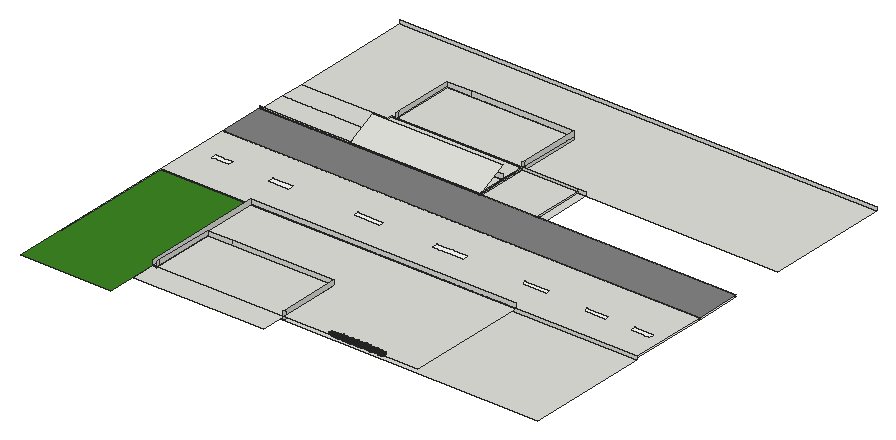
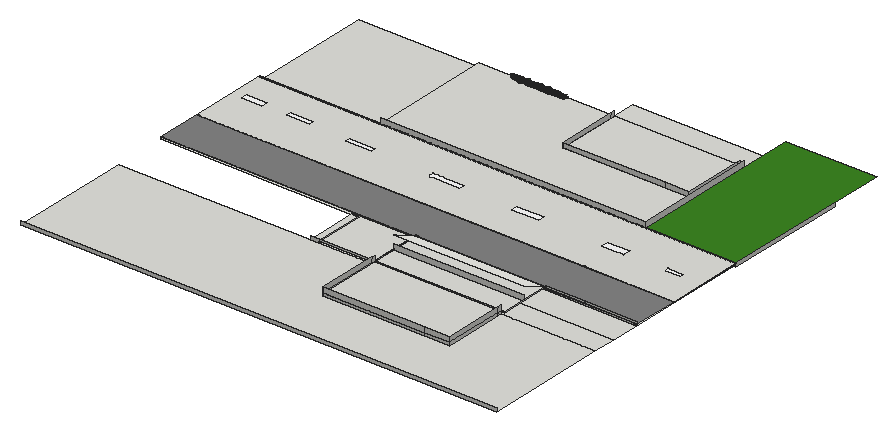
# SketchUp Ruby script. Lengths in inches.
U = 1.inch
M = Sketchup.active_model
def pt(a) = Geom::Point3d.new(a.map { |v| v * U })
def face(e, loops, mat)
  f = e.add_face(loops[0].map { |a| pt(a) })
  loops[1..].each { |l| e.add_face(l.map { |a| pt(a) }).erase! }
  f.material = f.back_material = mat if mat
  f
end
# faces: each face lists its corners as indices into pts; further lists are holes
def faces(e, pts, list, mat = nil) = list.each { |f| face(e, (f[0].is_a?(Array) ? f : [f]).map { |l| l.map { |i| pts[i] } }, mat) }
# xy, xz, yz: faces in a plane at the given z, y or x. An outline is a flat list of corners, or four numbers for a rectangle; further outlines are holes
def ring(l) = l.size == 4 ? [[l[0], l[1]], [l[2], l[1]], [l[2], l[3]], [l[0], l[3]]] : l.each_slice(2).to_a
def flat(e, list, mat, &to3) = list.each { |f| face(e, (f[0].is_a?(Array) ? f : [f]).map { |l| ring(l).map { |u, v| to3.(u, v) } }, mat) }
def xy(e, z, list, mat = nil) = flat(e, list, mat) { |x, y| [x, y, z] }
def xz(e, y, list, mat = nil) = flat(e, list, mat) { |x, z| [x, y, z] }
def yz(e, x, list, mat = nil) = flat(e, list, mat) { |y, z| [x, y, z] }
def lines(e, pts, list) = list.each { |a, b| e.add_line(pt(pts[a]), pt(pts[b])) }
# prism: a flat outline (further loops are holes) pulled along v
def prism(e, loops, v, mat = nil)
  f = face(e, loops, mat); d = Geom::Vector3d.new(v.map { |x| x * U })
  f.pushpull(f.normal.samedirection?(d) ? d.length : -d.length)
end
def box(e, o, s, mat = nil) = prism(e, [[o, [o[0] + s[0], o[1], o[2]], [o[0] + s[0], o[1] + s[1], o[2]], [o[0], o[1] + s[1], o[2]]]], [0, 0, s[2]], mat)
def at(x, y, z, deg = 0) = Geom::Transformation.translation(pt([x, y, z])) * Geom::Transformation.rotation(ORIGIN, Z_AXIS, deg.degrees)
def axes(o, x, y, z) = Geom::Transformation.new([*x, 0, *y, 0, *z, 0, *pt(o).to_a, 1])
def part(name) = M.definitions.add(name)
# library, detail: a bought-in or finely detailed component or shape, given as its bounding box
def library(name, o, s) = part(name).tap { |d| box(d.entities, o, s) }
def detail(e, o, s) = box(e.add_group.entities, o, s)
def put(e, d, t, mat = nil) = e.add_instance(d, t).tap { |i| i.material = mat if mat }
def group(e, t, mat = nil) = e.add_group.tap { |g| g.transformation = t; g.material = mat if mat }.entities
root = M.entities
M.materials.add("Color_3").color = [255, 255, 255]
M.materials.add("Material82").color = [68, 110, 58]
M.materials.add("Material83").color = [48, 90, 38]
M.materials.add("Material84").color = [68, 110, 48]
M.materials.add("Material85").color = [48, 90, 48]
M.materials.add("Material86").color = [58, 110, 58]
M.materials.add("Material87").color = [58, 90, 38]
M.materials.add("Material88").color = [68, 100, 58]
M.materials.add("Material89").color = [48, 100, 38]
M.materials.add("[Color M01]").color = [60, 133, 34]
M.materials.add("[Tile Grey]1").color = [132, 132, 132]
c1 = part("grass00")
p = [[-0.6875,0.15,0],[-0.56,0.08,5.52],[-0.04,0.03,2.76],[0.48,-0.02,0],[0.35,-0.02,5.52],[-0.1,-0.14,5.52],
  [-0.12,0.65,8.37],[-0.42,0.65,8.37]]
faces(c1.entities,p,[[0,1,2,3],[3,2,4],[1,5,2],[5,4,2],[1,6,5],[4,5,6],[7,6,1]])
c2 = part("Group16\#1")
put(c2.entities,c1,axes([1.44,-0.61,-0.01],[0.05352,0.12609,0],[-0.10704,0.04543,0.07239],[0.06664,-0.02828,0.11628]),"Material85")
put(c2.entities,c1,axes([0.76,-0.15,-0.01],[0.04676,0.24062,0],[-0.23162,0.04501,0.06642],[0.0652,-0.01267,0.23595]),"Material82")
put(c2.entities,c1,axes([0.79,0.01,-0.01],[-0.00606,0.34651,0],[-0.34381,-0.00602,0.0432],[0.04319,0.00076,0.34386]))
put(c2.entities,c1,axes([1,0.23,-0.01],[-0.07192,0.31144,0],[-0.28722,-0.06632,0.1236],[0.12043,0.02781,0.29478]),"Material84")
put(c2.entities,c1,axes([1.66,0.77,-0.01],[-0.13828,0.29651,0],[-0.21551,-0.1005,0.22471],[0.20365,0.09498,0.23779]),"Material89")
put(c2.entities,c1,axes([0.6875,0.52,-0.01],[-0.18126,0.24051,0],[-0.22746,-0.17142,0.09788],[0.07817,0.05891,0.28481]),"Material84")
put(c2.entities,c1,axes([0.68,0.78,-0.01],[-0.215,0.18688,0],[-0.12385,-0.14248,0.21334],[0.13995,0.16101,0.18878]),"Material82")
put(c2.entities,c1,axes([0.56,1,-0.01],[-0.13756,0.07624,0],[-0.06159,-0.11112,0.0927],[0.04494,0.08108,0.12705]),"Material84")
put(c2.entities,c1,axes([0.2,0.64,-0.01],[-0.23729,0.07254,0],[-0.05711,-0.18681,0.153],[0.04473,0.14632,0.19535]),"Material89")
put(c2.entities,c1,axes([0.0625,0.72,-0.01],[-0.28874,0.02525,0],[-0.02179,-0.24916,0.14647],[0.01276,0.14591,0.25012]),"Material82")
put(c2.entities,c1,axes([-0.08,0.62,-0.01],[-0.34089,-0.04187,0],[0.03255,-0.26504,0.216],[-0.02633,0.21439,0.26703]),"Material89")
put(c2.entities,c1,axes([-0.34,0.98,-0.01],[-0.14314,-0.0493,0],[0.04397,-0.12769,0.06843],[-0.02228,0.0647,0.13505]),"Material89")
put(c2.entities,c1,axes([-0.87,1.45,-0.01],[-0.23488,-0.14114,0],[0.13761,-0.22901,0.06087],[-0.03135,0.05217,0.26717]))
put(c2.entities,c1,axes([-0.72,0.77,-0.01],[-0.14208,-0.13251,0],[0.07209,-0.0773,0.16301],[-0.11118,0.11922,0.1057]),"Material89")
put(c2.entities,c1,axes([-0.62,0.43,-0.01],[-0.14845,-0.21203,0],[0.18654,-0.13061,0.12304],[-0.10079,0.07057,0.22772]),"Material82")
put(c2.entities,c1,axes([-0.68,0.29,-0.01],[-0.13639,-0.32136,0],[0.31723,-0.13464,0.05579],[-0.05136,0.0218,0.34462]),"Material83")
put(c2.entities,c1,axes([-0.64,0.125,-0.01],[-0.0458,-0.23569,0],[0.22124,-0.043,0.08276],[-0.08124,0.01579,0.22538]),"Material86")
put(c2.entities,c1,axes([-1.6,-0.03,-0.01],[0.00576,-0.32897,0],[0.27526,0.00482,0.18018],[-0.18015,-0.00315,0.2753]),"Material84")
put(c2.entities,c1,axes([-1.36,-0.31,-0.01],[0.05718,-0.24765,0],[0.18172,0.04196,0.17267],[-0.16825,-0.03885,0.1865]),"Material89")
put(c2.entities,c1,axes([-1.54,-0.72,-0.01],[0.06537,-0.14017,0],[0.13555,0.06321,0.03939],[-0.0357,-0.01665,0.14956]))
put(c2.entities,c1,axes([-1.19,-0.9,-0.01],[0.09597,-0.12735,0],[0.11214,0.08451,0.07557],[-0.06035,-0.04548,0.14042]),"Material88")
put(c2.entities,c1,axes([-0.47,-0.54,-0.01],[0.11588,-0.10072,0],[0.0618,0.0711,0.12124],[-0.07953,-0.0915,0.0942]))
put(c2.entities,c1,axes([-0.47,-0.84,-0.01],[0.11927,-0.0661,0],[0.06603,0.11913,0.00646],[-0.00313,-0.00565,0.13621]),"Material84")
put(c2.entities,c1,axes([-0.38,-1.24,-0.01],[0.28037,-0.08571,0],[0.0618,0.20215,0.20315],[-0.05939,-0.19428,0.21139]),"Material88")
put(c2.entities,c1,axes([-0.06,-0.66,-0.01],[0.22719,-0.01987,0],[0.01247,0.14255,0.17758],[-0.01547,-0.17691,0.1431]),"Material87")
put(c2.entities,c1,axes([0.11,-0.89,-0.01],[0.14882,0.01828,0],[-0.01058,0.08611,0.12229],[0.01491,-0.12138,0.08676]),"Material85")
put(c2.entities,c1,axes([0.25,-0.72,-0.01],[0.20481,0.07053,0],[-0.06206,0.18022,0.10291],[0.03351,-0.0973,0.1906]),"Material85")
put(c2.entities,c1,axes([0.85,-1.42,-0.01],[0.16481,0.09904,0],[-0.09472,0.15762,0.05616],[0.02893,-0.04814,0.18389]),"Material84")
put(c2.entities,c1,axes([1.01,-1.09,-0.01],[0.21858,0.20385,0],[-0.17495,0.1876,0.15339],[0.10462,-0.11218,0.25652]),"Material89")
put(c2.entities,c1,axes([1.01,-0.71,-0.01],[0.08733,0.12473,0],[-0.06445,0.04512,0.13037],[0.1068,-0.07477,0.07867]),"Material85")
c3 = part("Group15\#1")
put(c3.entities,c2,at(0,0,0))
c4 = part("3darcstudiotree_grass00\#1")
put(c4.entities,c3,at(0,0,0))
c5 = part("Untitled (5)")
xy(c5.entities,0,[[[158.81,26.5625,306.06,993.3125],[226.57,518.17,239.57,583.92],[225.28,357.51,237.28,411.51],[222.61,182.28,236.36,226.53],[239.71,931.55,251.46,972.3],[233.64,703.93,242.14,755.18],[240.05,835.03,248.8,880.53],[222.04,66.5,231.29,100.5]]])
xy(c5.entities,0,[[222.04,66.5,231.29,100.5],[222.61,182.28,236.36,226.53],[225.28,357.51,237.28,411.51],[226.57,518.17,239.57,583.92],[233.64,703.93,242.14,755.18],
  [240.05,835.03,248.8,880.53],[239.71,931.55,251.46,972.3]],"Color_3")
xy(root,-42.1875,[[1048.66,387.84,1048.66,659.09,2096.97,659.09,2096.97,387.84,1534.73,387.84,1534.73,528.53,1257.22,528.53,1257.22,387.84],[1257.22,387.84,1534.73,528.53]])
xy(root,-37.75,[[1048.3125,660.69,2096.625,831.37],[1048.3125,831.37,1248,932.5],[1248,831.37,1248,932.5,1534.38,932.5,1534.38,1046.93,1657.0625,1046.93,1657.0625,932.5,2096.625,932.5,2096.625,831.37],[1048.3125,932.5,1534.38,994.94],[1657.0625,932.5,1674.65,1046.93],
  [1048.3125,994.94,1534.38,1046.93],[1048.3125,1046.93,1048.3125,1318.18,2096.625,1318.18,2096.625,1046.93,1534.38,1046.93,1534.38,1187.62,1256.88,1187.62,1256.88,1046.93],[1256.88,1046.93,1534.38,1187.62]])
xy(root,-35.625,[[1248.34,335.84,1534.73,335.84,1534.73,528.53,1257.22,528.53,1257.22,387.84,1248.34,387.84]])
xy(root,-34.75,[[1048.3125,660.69,2096.625,831.37]])
xy(root,-34.6875,[[1534.38,932.5,1657.0625,1046.93]])
xy(root,-34.17,[[1248.34,387.84,1831.09,659.09]])
xy(root,-34.17,[[1048.66,273.53,1248.34,659.09]],"[Color M01]")
xy(root,-34.17,[[1048.3125,831.37,2096.625,932.5]],"[Tile Grey]1")
xy(root,-33.625,[[1048.3125,932.5,1163.9375,932.62],[1163.9375,932.5,1534.38,932.62]])
xy(root,-31.1875,[[1248,932.5,1534.38,932.62],[1248,932.62,1534.38,994.94],[1248,994.94,1534.38,994.94,1534.38,1187.62,1256.88,1187.62,1256.88,1046.93,1248,1046.93]])
xz(root,528.53,[[1257.22,-42.1875,1311.1,-35.625],[1311.1,-42.1875,1534.73,-35.625],[1257.22,-35.625,1311.1,-24.25],[1311.1,-35.625,1534.73,-24.25]])
xz(root,659.09,[[1048.66,-42.1875,2096.97,-34.17],[1248.34,-34.17,1831.09,-22.8]])
xz(root,660.69,[[1048.3125,-37.75,2096.625,-34.75]])
xz(root,831.37,[[1048.3125,-37.75,1248,-34.75],[1248,-37.75,2096.625,-34.75],[1048.3125,-34.75,1248,-34.17],[1248,-34.75,2096.625,-34.17]])
xz(root,932.5,[[1048.3125,-37.75,1248,-34.17],[1248,-37.75,1534.38,-34.6875],[1657.0625,-37.75,1674.65,-34.6875],[1248,-34.6875,1534.38,-34.17],[1534.38,-34.6875,1657.0625,-34.17],
  [1657.0625,-34.6875,1674.65,-34.17],[1048.3125,-34.17,1534.38,-33.75],[1534.38,-34.17,1657.0625,-33.75],[1657.0625,-34.17,1674.65,-33.75],[1048.3125,-33.75,1534.38,-33.625],
  [1534.38,-33.75,2096.625,-33.42],[1163.9375,-33.625,1534.38,-33.625,1534.38,-31.1875,1248,-31.1875,1248,-29.74,1163.9375,-29.74]])
xz(root,932.62,[[1048.3125,-33.625,1163.9375,-29.74],[1163.9375,-33.625,1163.9375,-29.74,1248,-29.74,1248,-31.1875,1534.38,-31.1875,1534.38,-33.625]])
xz(root,994.94,[[1248,-31.1875,1534.38,-19.8125]])
xz(root,1046.93,[[1256.88,-37.75,1534.38,-29.74],[1657.0625,-37.75,1674.65,-29.74],[1534.38,-34.6875,1657.0625,-29.74],[1248,-31.1875,1256.88,-29.74]])
xz(root,1187.62,[[1256.88,-37.75,1310.75,-31.1875],[1310.75,-37.75,1534.38,-31.1875],[1256.88,-31.1875,1310.75,-19.8125],[1310.75,-31.1875,1534.38,-19.8125]])
xz(root,1318.18,[[1048.3125,-37.75,2096.625,-29.74]])
yz(root,1048.66,[[387.84,-42.1875,659.09,-34.17]])
yz(root,1163.9375,[[932.5,-33.625,932.62,-29.74]])
yz(root,1248,[[932.5,-31.1875,932.62,-31.13,932.62,-29.74,932.5,-29.74],[932.5,-31.1875,932.62,-31.1875,932.62,-31.13],[932.62,-31.1875,932.62,-31.13,935.62,-29.74,994.94,-29.74,994.94,-31.1875],[994.94,-31.1875,1046.93,-29.74],[932.62,-31.13,935.62,-29.74,932.62,-29.74]])
yz(root,1248.34,[[387.84,-34.17,659.09,-22.8]])
yz(root,1256.88,[[1046.93,-37.75,1054,-31.1875],[1054,-37.75,1187.62,-31.1875],[1046.93,-31.1875,1054,-19.8125],[1054,-31.1875,1187.62,-19.8125]])
yz(root,1257.22,[[387.84,-42.1875,394.91,-35.625],[394.91,-42.1875,528.53,-35.625],[387.84,-35.625,394.91,-24.25],[394.91,-35.625,528.53,-24.25]])
yz(root,1534.38,[[932.5,-37.75,994.94,-34.6875],[994.94,-37.75,1022.06,-34.6875],[1022.06,-37.75,1023.55,-34.6875],[1023.55,-37.75,1046.93,-34.6875],[1046.93,-37.75,1054,-31.1875],
  [1054,-37.75,1187.62,-31.1875],[932.5,-34.6875,932.5,-33.625,932.62,-33.625,932.62,-31.1875,994.94,-31.1875,994.94,-34.6875],[994.94,-34.6875,1022.06,-31.1875],[1022.06,-34.6875,1023.55,-31.1875],[1023.55,-34.6875,1046.93,-31.1875],
  [932.5,-33.625,932.62,-33.42],[932.5,-33.42,932.62,-32.8],[932.5,-32.8,932.62,-31.1875],[932.5,-31.1875,932.5,-29.74,935.62,-29.74],[932.5,-31.1875,994.94,-31.1875,994.94,-29.74,935.62,-29.74],
  [994.94,-31.1875,1022.06,-29.74],[1022.06,-31.1875,1023.55,-29.74],[1023.55,-31.1875,1046.93,-29.74],[1046.93,-31.1875,1054,-19.8125],[1054,-31.1875,1187.62,-19.8125]])
yz(root,1534.73,[[387.84,-42.1875,394.91,-35.625],[394.91,-42.1875,528.53,-35.625],[387.84,-35.625,394.91,-24.25],[394.91,-35.625,528.53,-24.25]])
yz(root,1657.0625,[[932.5,-37.75,1046.93,-34.6875]])
p = [[1248,994.94,-2.1875],[1248,935.62,-29.74],[1248,932.62,-31.13],[1248,932.5,-31.1875],[1534.38,932.5,-31.1875],[1534.38,935.62,-29.74],
  [1534.38,994.94,-2.1875]]
faces(root,p,[[0,1,2,3,4,5,6]])
put(root,c4,axes([1681.51,387.7,-34.17],[-4.17606,0.09309,0],[-0.21865,-1.52546,-0.00256],[-0.00085,-0.00591,1.70382]))
put(root,c4,axes([1672.63,388.31,-34.17],[0.26998,-1.38938,0],[4.08981,0.1236,-0.05496],[0.34231,0.01035,1.9204]))
put(root,c4,axes([1731.29,387.97,-34.17],[-3.32048,-0.89448,0],[2.67505,-1.54445,-0.03279],[0.08824,-0.05095,1.69581]))
put(root,c4,axes([1751.17,387.88,-34.17],[-2.85085,-0.66888,0],[2.41654,-1.60188,-0.00321],[0.00686,-0.00455,1.48019]))
put(root,c4,axes([1657.76,388.31,-34.17],[3.43516,0.20919,0],[-0.57575,1.47043,-0.03647],[-0.03089,0.0789,1.56991]))
put(root,c4,axes([1706.98,388.41,-34.17],[-3.1613,-1.38915,0],[3.20855,-1.13563,-0.02493],[0.08224,-0.02911,1.43253]))
put(root,c4,axes([1728.26,388.5,-34.17],[-2.12705,-1.09895,0],[2.82257,-0.84968,-0.04177],[0.17079,-0.05141,1.36919]))
put(root,c4,axes([1686.96,388.45,-34.17],[-3.25209,-0.85971,0],[2.35344,-1.3846,-0.05337],[0.14871,-0.08749,1.58535]))
put(root,c4,axes([1701.65,388.66,-34.17],[-2.22741,-1.08823,0],[2.74712,-0.87452,-0.02577],[0.11865,-0.03777,1.56591]))
put(root,c4,axes([1693.98,388.41,-34.17],[-3.60513,-0.15499,0],[0.46196,-1.67121,-0.01401],[0.00822,-0.02974,1.72979]))
put(root,c4,axes([1705.29,389.55,-34.17],[2.77032,-1.11765,0],[2.79461,1.07735,-0.00015],[0.00071,0.00027,1.98495]))
put(root,c4,axes([1701.52,389.375,-34.17],[-2.63384,-1.55649,0],[3.02127,-0.79514,-0.04802],[0.24921,-0.06559,1.69851]))
put(root,c4,axes([1683.08,389.46,-34.17],[-0.69591,-1.28996,0],[3.84518,-0.32263,-0.04713],[0.24772,-0.02078,1.58351]))
put(root,c4,axes([1696.41,389.5625,-34.17],[4.30833,-0.24109,0],[0.6166,1.71371,-0.05794],[0.04515,0.12549,1.82474]))
put(root,c4,axes([1679.21,390.01,-34.17],[3.37733,-0.03199,0],[0.10215,1.67739,-0.04057],[0.00409,0.06713,1.33829]))
put(root,c4,axes([1646.57,389.47,-34.17],[-2.59394,1.01102,0],[-3.072,-1.22583,-0.01852],[-0.05979,-0.02386,1.50457]))
put(root,c4,axes([1665.19,390.41,-34.17],[2.33818,-1.41789,0],[2.84176,0.72884,-0.04791],[0.27889,0.07153,1.76421]))
put(root,c4,axes([1670.8125,390.47,-34.17],[0.86182,-1.33711,0],[3.4036,0.34119,-0.00558],[0.03445,0.00345,1.6757]))
put(root,c4,axes([1751.01,390.18,-34.17],[2.4354,1.06288,0],[-2.86607,1.02137,-0.0306],[-0.14622,0.05211,1.86488]))
put(root,c4,axes([1715.03,390.06,-34.17],[0.39811,1.50692,0],[-3.94981,0.16229,-0.02993],[-0.16157,0.00664,1.61572]))
put(root,c4,axes([1738.09,390.23,-34.17],[-3.73597,-0.76469,0],[1.79369,-1.36294,-0.02416],[0.05526,-0.04199,1.4491]))
put(root,c4,axes([1662.6,390.27,-34.17],[-3.25297,-0.61029,0],[1.91072,-1.58399,-0.03826],[0.09019,-0.07477,1.82966]))
put(root,c4,axes([1711.27,390.8,-34.17],[3.60935,-0.56815,0],[1.37625,1.35979,-0.02611],[0.05001,0.04941,1.43783]))
put(root,c4,axes([1652.21,390.22,-34.17],[-2.1063,1.53486,0],[-3.86767,-0.82549,-0.04902],[-0.23106,-0.04932,1.76654]))
put(root,c4,axes([1743,390.64,-34.17],[-2.95598,-0.91326,0],[2.43781,-1.22721,-0.04081],[0.12436,-0.0626,1.46417]))
put(root,c4,axes([1688.03,390.83,-34.17],[-3.50198,-0.71469,0],[1.86103,-1.41828,-0.02021],[0.05866,-0.0447,1.91641]))
put(root,c4,axes([1728.25,390.74,-34.17],[-0.65253,1.4678,0],[-3.82967,-0.26479,-0.02601],[-0.14603,-0.0101,1.66111]))
put(root,c4,axes([1654.59,390.73,-34.17],[-1.7142,1.30326,0],[-3.68982,-0.75483,-0.04385],[-0.17675,-0.03616,1.41492]))
put(root,c4,axes([1720.28,390.83,-34.17],[-4.08637,0.5893,0],[-1.1512,-1.24155,-0.04181],[-0.0785,-0.08466,1.37365]))
put(root,c4,axes([1731.76,390.93,-34.17],[0.62564,1.8219,0],[-4.46763,0.23861,-0.03426],[-0.17796,0.0095,1.77113]))
put(root,c4,axes([1662.43,391.67,-34.17],[2.39,-1.25303,0],[3.55352,1.05416,-0.05537],[0.20037,0.05944,1.50911]))
put(root,c4,axes([1728.1,391.57,-34.17],[3.95759,-0.11816,0],[0.2883,1.50178,-0.04662],[0.02067,0.10765,1.68074]))
put(root,c4,axes([1701.19,391.82,-34.17],[2.75838,0.79761,0],[-2.27657,1.22449,-0.01003],[-0.02813,0.01513,1.36834]))
put(root,c4,axes([1749.37,392.06,-34.17],[0.25727,-1.4604,0],[3.98489,0.10918,-0.0172],[0.09613,0.00263,1.67763]))
put(root,c4,axes([1694.32,391.5625,-34.17],[-1.99433,1.44629,0],[-3.30766,-0.70937,-0.03157],[-0.17706,-0.03797,1.80167]))
put(root,c4,axes([1715.92,391.72,-34.17],[0.18137,1.61713,0],[-3.86456,0.06741,-0.03464],[-0.18684,0.00326,1.56527]))
put(root,c4,axes([1689.79,392.26,-34.17],[3.4743,0.19553,0],[-0.61359,1.69568,-0.03434],[-0.02545,0.07034,1.70799]))
put(root,c4,axes([1733.76,391.64,-34.17],[-2.17573,1.65884,0],[-3.97455,-0.81077,-0.04288],[-0.19169,-0.0391,1.68813]))
put(root,c4,axes([1666.86,391.89,-34.17],[-1.73323,1.28831,0],[-3.70175,-0.77456,-0.05129],[-0.19346,-0.04048,1.34106]))
put(root,c4,axes([1684,391.87,-34.17],[-4.09244,0.60833,0],[-1.31907,-1.38013,-0.00238],[-0.00395,-0.00413,1.31717]))
put(root,c4,axes([1743.56,392.57,-34.17],[-0.4279,-1.35562,0],[4.45161,-0.21854,-0.05859],[0.31746,-0.01559,1.83593]))
put(root,c4,axes([1723.24,392.16,-34.17],[-4.63629,0.17249,0],[-0.31305,-1.3087,-0.02738],[-0.01684,-0.0704,1.63584]))
put(root,c4,axes([1657.71,392.67,-34.17],[-1.23898,-1.77649,0],[4.18164,-0.45359,-0.02011],[0.11729,-0.01272,1.9663]))
put(root,c4,axes([1706.72,392.46,-34.17],[-4.11217,-0.39094,0],[0.86082,-1.40827,-0.01967],[0.02693,-0.04406,1.60841]))
put(root,c4,axes([1737.51,392.9375,-34.17],[3.58477,-0.09461,0],[0.24683,1.45461,-0.02393],[0.00869,0.05119,1.50627]))
put(root,c4,axes([1650.37,392.72,-34.17],[-2.67553,-0.98375,0],[2.79136,-1.18074,-0.04642],[0.15585,-0.06593,1.51042]))
put(root,c4,axes([1645.9,392.39,-34.17],[-1.47744,1.354,0],[-3.50661,-0.5951,-0.01574],[-0.08407,-0.01427,1.66349]))
put(root,c4,axes([1709.86,392.99,-34.17],[-0.90047,-1.75818,0],[4.05941,-0.32336,-0.03802],[0.21461,-0.0171,1.78771]))
put(root,c4,axes([1671.14,392.71,-34.17],[-1.19077,1.57344,0],[-3.27951,-0.38601,-0.00408],[-0.02113,-0.00249,1.38631]))
put(root,c4,axes([1677.81,392.99,-34.17],[1.23256,1.36805,0],[-3.36714,0.47182,-0.0026],[-0.01342,0.00188,1.46428]))
put(root,c4,axes([1715.7,393.86,-34.17],[2.68425,0.98126,0],[-3.08103,1.31083,-0.0132],[-0.04194,0.01784,1.58767]))
put(root,c4,axes([1687.64,394.0625,-34.17],[2.94498,0.60485,0],[-2.04543,1.54892,-0.0178],[-0.03241,0.02454,1.30843]))
put(root,c4,axes([1660.15,393.84,-34.17],[-3.78694,0.18795,0],[-0.43899,-1.37568,-0.01354],[-0.00909,-0.02849,1.41676]))
put(root,c4,axes([1734.8,394.19,-34.17],[1.29207,1.70529,0],[-3.1938,0.37636,-0.01522],[-0.08109,0.00956,1.38916]))
put(root,c4,axes([1672.93,394.45,-34.17],[-2.41696,-1.08887,0],[3.39352,-1.17154,-0.03006],[0.11594,-0.04003,1.73276]))
put(root,c4,axes([1709.29,394.24,-34.17],[-3.99047,-0.40873,0],[1.06863,-1.62266,-0.00758],[0.01027,-0.0156,1.7185]))
put(root,c4,axes([1699.07,394.29,-34.17],[-4.3017,0.59676,0],[-1.104,-1.2377,-0.00518],[-0.01285,-0.0144,1.86492]))
put(root,c5,axes([1019.84,1017.18,-34.17],[0,-1.17,0],[1.0847,0,0],[0,0,1]))
